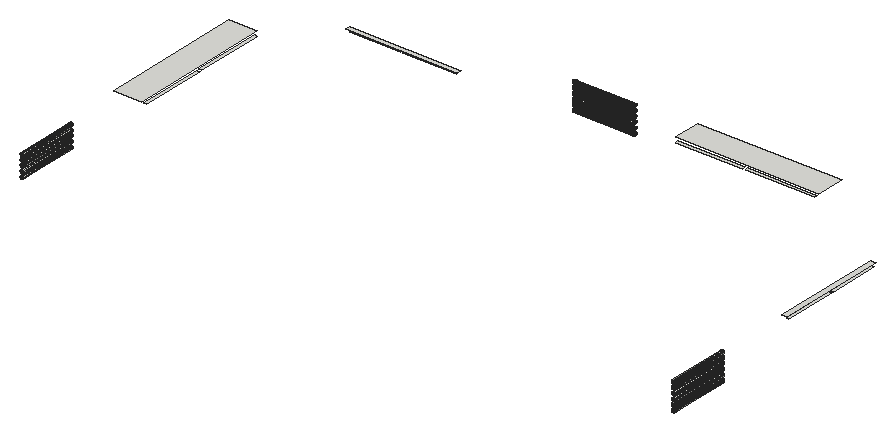
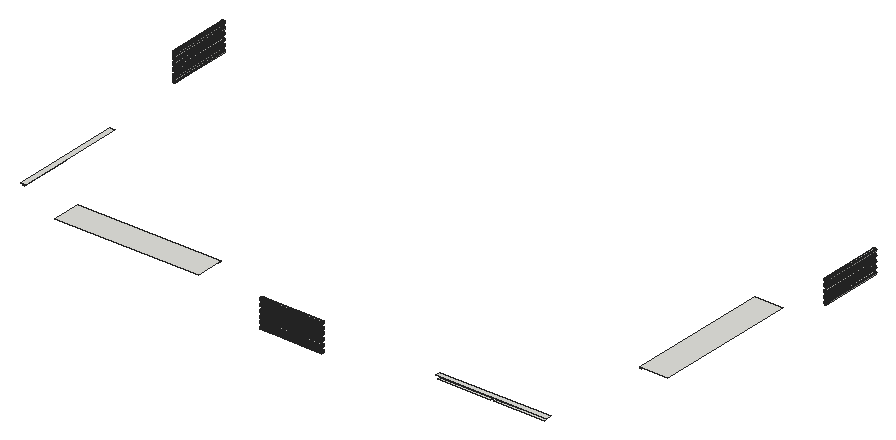
# SketchUp Ruby script. Lengths in inches.
U = 1.inch
M = Sketchup.active_model
def pt(a) = Geom::Point3d.new(a.map { |v| v * U })
def face(e, loops, mat)
  f = e.add_face(loops[0].map { |a| pt(a) })
  loops[1..].each { |l| e.add_face(l.map { |a| pt(a) }).erase! }
  f.material = f.back_material = mat if mat
  f
end
# faces: each face lists its corners as indices into pts; further lists are holes
def faces(e, pts, list, mat = nil) = list.each { |f| face(e, (f[0].is_a?(Array) ? f : [f]).map { |l| l.map { |i| pts[i] } }, mat) }
# xy, xz, yz: faces in a plane at the given z, y or x. An outline is a flat list of corners, or four numbers for a rectangle; further outlines are holes
def ring(l) = l.size == 4 ? [[l[0], l[1]], [l[2], l[1]], [l[2], l[3]], [l[0], l[3]]] : l.each_slice(2).to_a
def flat(e, list, mat, &to3) = list.each { |f| face(e, (f[0].is_a?(Array) ? f : [f]).map { |l| ring(l).map { |u, v| to3.(u, v) } }, mat) }
def xy(e, z, list, mat = nil) = flat(e, list, mat) { |x, y| [x, y, z] }
def xz(e, y, list, mat = nil) = flat(e, list, mat) { |x, z| [x, y, z] }
def yz(e, x, list, mat = nil) = flat(e, list, mat) { |y, z| [x, y, z] }
def lines(e, pts, list) = list.each { |a, b| e.add_line(pt(pts[a]), pt(pts[b])) }
# prism: a flat outline (further loops are holes) pulled along v
def prism(e, loops, v, mat = nil)
  f = face(e, loops, mat); d = Geom::Vector3d.new(v.map { |x| x * U })
  f.pushpull(f.normal.samedirection?(d) ? d.length : -d.length)
end
def box(e, o, s, mat = nil) = prism(e, [[o, [o[0] + s[0], o[1], o[2]], [o[0] + s[0], o[1] + s[1], o[2]], [o[0], o[1] + s[1], o[2]]]], [0, 0, s[2]], mat)
def at(x, y, z, deg = 0) = Geom::Transformation.translation(pt([x, y, z])) * Geom::Transformation.rotation(ORIGIN, Z_AXIS, deg.degrees)
def axes(o, x, y, z) = Geom::Transformation.new([*x, 0, *y, 0, *z, 0, *pt(o).to_a, 1])
def part(name) = M.definitions.add(name)
# library, detail: a bought-in or finely detailed component or shape, given as its bounding box
def library(name, o, s) = part(name).tap { |d| box(d.entities, o, s) }
def detail(e, o, s) = box(e.add_group.entities, o, s)
def put(e, d, t, mat = nil) = e.add_instance(d, t).tap { |i| i.material = mat if mat }
def group(e, t, mat = nil) = e.add_group.tap { |g| g.transformation = t; g.material = mat if mat }.entities
root = M.entities
xy(root,647.61,[[1494,1126.01,1500,1249.86],[1494,1255.86,1500,1373.7],[211.11,1458.8125,328.96,1464.8125],[334.96,1458.8125,458.8,1464.8125]])
xy(root,653.61,[[1488,1120.01,1500,1379.7],[205.11,1452.8125,464.8,1464.8125]])
xy(root,696.625,[[138,949.59,144,1104.875],[138,1110.875,144,1272.16],[984.78,1440.8125,1140.0625,1446.8125],[1146.0625,1440.8125,1307.35,1446.8125]])
xy(root,702.625,[[72,943.59,138,1278.16],[978.78,1446.8125,1313.35,1512.8125]])
p = [[1535.52,886.83,633.14],[1536.47,886.83,633.02],[1536.47,743.45,633.02],[1535.52,743.45,633.14],[1537.43,886.83,633.14],[1537.43,743.45,633.14],
  [697.99,1500.33,633.14],[697.99,1501.28,633.02],[841.36,1501.28,633.02],[841.36,1500.33,633.14],[697.99,1502.24,633.14],[841.36,1502.24,633.14],
  [1534.63,886.83,633.51],[1534.63,743.45,633.51],[1538.32,886.83,633.51],[1538.32,743.45,633.51],[697.99,1499.44,633.51],[841.36,1499.44,633.51],
  [697.99,1503.13,633.51],[841.36,1503.13,633.51],[1533.87,886.83,634.1],[1533.87,743.45,634.1],[1539.08,886.83,634.1],[1539.08,743.45,634.1],
  [697.99,1498.68,634.1],[841.36,1498.68,634.1],[697.99,1503.89,634.1],[841.36,1503.89,634.1],[1533.28,886.83,634.86],[1533.28,743.45,634.86],
  [1539.67,886.83,634.86],[1539.67,743.45,634.86],[697.99,1498.09,634.86],[841.36,1498.09,634.86],[697.99,1504.48,634.86],[841.36,1504.48,634.86],
  [1532.91,886.83,635.75],[1532.91,743.45,635.75],[1540.03,886.83,635.75],[1540.03,743.45,635.75],[697.99,1497.72,635.75],[841.36,1497.72,635.75],
  [697.99,1504.85,635.75],[841.36,1504.85,635.75],[1532.79,886.83,636.7],[1532.79,743.45,636.7],[1540.16,886.83,636.7],[1540.16,743.45,636.7],
  [697.99,1497.6,636.7],[841.36,1497.6,636.7],[697.99,1504.97,636.7],[841.36,1504.97,636.7],[1532.91,886.83,637.66],[1532.91,743.45,637.66],
  [1540.03,886.83,637.66],[1540.03,743.45,637.66],[697.99,1497.72,637.66],[841.36,1497.72,637.66],[697.99,1504.85,637.66],[841.36,1504.85,637.66],
  [1533.28,886.83,638.55],[1533.28,743.45,638.55],[1539.67,886.83,638.55],[1539.67,743.45,638.55],[697.99,1498.09,638.55],[841.36,1498.09,638.55],
  [697.99,1504.48,638.55],[841.36,1504.48,638.55],[1533.87,886.83,639.3125],[1533.87,743.45,639.3125],[1539.08,886.83,639.3125],[1539.08,743.45,639.3125],
  [697.99,1498.68,639.3125],[841.36,1498.68,639.3125],[697.99,1503.89,639.3125],[841.36,1503.89,639.3125],[1534.63,886.83,639.9],[1534.63,743.45,639.9],
  [1538.32,886.83,639.9],[1538.32,743.45,639.9],[697.99,1499.44,639.9],[841.36,1499.44,639.9],[697.99,1503.13,639.9],[841.36,1503.13,639.9],
  [1535.52,886.83,640.27],[1535.52,743.45,640.27],[1537.43,886.83,640.27],[1537.43,743.45,640.27],[697.99,1500.33,640.27],[841.36,1500.33,640.27],
  [697.99,1502.24,640.27],[841.36,1502.24,640.27],[1536.47,886.83,640.39],[1536.47,743.45,640.39],[697.99,1501.28,640.39],[841.36,1501.28,640.39],
  [83.53,662.8,645.02],[82.57,662.8,645.14],[82.57,806.17,645.14],[83.53,806.17,645.02],[84.48,662.8,645.14],[84.48,806.17,645.14],
  [1535.52,886.83,645.14],[1536.47,886.83,645.02],[1536.47,743.45,645.02],[1535.52,743.45,645.14],[1537.43,886.83,645.14],[1537.43,743.45,645.14],
  [697.99,1500.33,645.14],[697.99,1501.28,645.02],[841.36,1501.28,645.02],[841.36,1500.33,645.14],[697.99,1502.24,645.14],[841.36,1502.24,645.14],
  [81.68,662.8,645.51],[81.68,806.17,645.51],[85.37,662.8,645.51],[85.37,806.17,645.51],[1534.63,886.83,645.51],[1534.63,743.45,645.51],
  [1538.32,886.83,645.51],[1538.32,743.45,645.51],[697.99,1499.44,645.51],[841.36,1499.44,645.51],[697.99,1503.13,645.51],[841.36,1503.13,645.51],
  [80.92,662.8,646.1],[80.92,806.17,646.1],[86.13,662.8,646.1],[86.13,806.17,646.1],[1533.87,886.83,646.1],[1533.87,743.45,646.1],
  [1539.08,886.83,646.1],[1539.08,743.45,646.1],[697.99,1498.68,646.1],[841.36,1498.68,646.1],[697.99,1503.89,646.1],[841.36,1503.89,646.1],
  [80.33,662.8,646.86],[80.33,806.17,646.86],[86.72,662.8,646.86],[86.72,806.17,646.86],[1533.28,886.83,646.86],[1533.28,743.45,646.86],
  [1539.67,886.83,646.86],[1539.67,743.45,646.86],[697.99,1498.09,646.86],[841.36,1498.09,646.86],[697.99,1504.48,646.86],[841.36,1504.48,646.86],
  [79.97,662.8,647.75],[79.97,806.17,647.75],[87.09,662.8,647.75],[87.09,806.17,647.75],[1532.91,886.83,647.75],[1532.91,743.45,647.75],
  [1540.03,886.83,647.75],[1540.03,743.45,647.75],[697.99,1497.72,647.75],[841.36,1497.72,647.75],[697.99,1504.85,647.75],[841.36,1504.85,647.75],
  [79.84,662.8,648.7],[79.84,806.17,648.7],[87.21,662.8,648.7],[87.21,806.17,648.7],[1532.79,886.83,648.7],[1532.79,743.45,648.7],
  [1540.16,886.83,648.7],[1540.16,743.45,648.7],[697.99,1497.6,648.7],[841.36,1497.6,648.7],[697.99,1504.97,648.7],[841.36,1504.97,648.7],
  [79.97,662.8,649.66],[79.97,806.17,649.66],[87.09,662.8,649.66],[87.09,806.17,649.66],[1532.91,886.83,649.66],[1532.91,743.45,649.66],
  [1540.03,886.83,649.66],[1540.03,743.45,649.66],[697.99,1497.72,649.66],[841.36,1497.72,649.66],[697.99,1504.85,649.66],[841.36,1504.85,649.66],
  [80.33,662.8,650.55],[80.33,806.17,650.55],[86.72,662.8,650.55],[86.72,806.17,650.55],[1533.28,886.83,650.55],[1533.28,743.45,650.55],
  [1539.67,886.83,650.55],[1539.67,743.45,650.55],[697.99,1498.09,650.55],[841.36,1498.09,650.55],[697.99,1504.48,650.55],[841.36,1504.48,650.55],
  [80.92,662.8,651.3125],[80.92,806.17,651.3125],[86.13,662.8,651.3125],[86.13,806.17,651.3125],[1533.87,886.83,651.3125],[1533.87,743.45,651.3125],
  [1539.08,886.83,651.3125],[1539.08,743.45,651.3125],[697.99,1498.68,651.3125],[841.36,1498.68,651.3125],[697.99,1503.89,651.3125],[841.36,1503.89,651.3125],
  [81.68,662.8,651.9],[81.68,806.17,651.9],[85.37,662.8,651.9],[85.37,806.17,651.9],[1534.63,886.83,651.9],[1534.63,743.45,651.9],
  [1538.32,886.83,651.9],[1538.32,743.45,651.9],[697.99,1499.44,651.9],[841.36,1499.44,651.9],[697.99,1503.13,651.9],[841.36,1503.13,651.9],
  [82.57,662.8,652.27],[82.57,806.17,652.27],[84.48,662.8,652.27],[84.48,806.17,652.27],[1535.52,886.83,652.27],[1535.52,743.45,652.27],
  [1537.43,886.83,652.27],[1537.43,743.45,652.27],[697.99,1500.33,652.27],[841.36,1500.33,652.27],[697.99,1502.24,652.27],[841.36,1502.24,652.27],
  [83.53,662.8,652.39],[83.53,806.17,652.39],[1536.47,886.83,652.39],[1536.47,743.45,652.39],[697.99,1501.28,652.39],[841.36,1501.28,652.39],
  [83.53,662.8,657.02],[82.57,662.8,657.14],[82.57,806.17,657.14],[83.53,806.17,657.02],[84.48,662.8,657.14],[84.48,806.17,657.14],
  [1535.52,886.83,657.14],[1536.47,886.83,657.02],[1536.47,743.45,657.02],[1535.52,743.45,657.14],[1537.43,886.83,657.14],[1537.43,743.45,657.14],
  [697.99,1500.33,657.14],[697.99,1501.28,657.02],[841.36,1501.28,657.02],[841.36,1500.33,657.14],[697.99,1502.24,657.14],[841.36,1502.24,657.14],
  [81.68,662.8,657.51],[81.68,806.17,657.51],[85.37,662.8,657.51],[85.37,806.17,657.51],[1534.63,886.83,657.51],[1534.63,743.45,657.51],
  [1538.32,886.83,657.51],[1538.32,743.45,657.51],[697.99,1499.44,657.51],[841.36,1499.44,657.51],[697.99,1503.13,657.51],[841.36,1503.13,657.51],
  [80.92,662.8,658.1],[80.92,806.17,658.1],[86.13,662.8,658.1],[86.13,806.17,658.1],[1533.87,886.83,658.1],[1533.87,743.45,658.1],
  [1539.08,886.83,658.1],[1539.08,743.45,658.1],[697.99,1498.68,658.1],[841.36,1498.68,658.1],[697.99,1503.89,658.1],[841.36,1503.89,658.1],
  [80.33,662.8,658.86],[80.33,806.17,658.86],[86.72,662.8,658.86],[86.72,806.17,658.86],[1533.28,886.83,658.86],[1533.28,743.45,658.86],
  [1539.67,886.83,658.86],[1539.67,743.45,658.86],[697.99,1498.09,658.86],[841.36,1498.09,658.86],[697.99,1504.48,658.86],[841.36,1504.48,658.86],
  [79.97,662.8,659.75],[79.97,806.17,659.75],[87.09,662.8,659.75],[87.09,806.17,659.75],[1532.91,886.83,659.75],[1532.91,743.45,659.75],
  [1540.03,886.83,659.75],[1540.03,743.45,659.75],[697.99,1497.72,659.75],[841.36,1497.72,659.75],[697.99,1504.85,659.75],[841.36,1504.85,659.75],
  [79.84,662.8,660.7],[79.84,806.17,660.7],[87.21,662.8,660.7],[87.21,806.17,660.7],[1532.79,886.83,660.7],[1532.79,743.45,660.7],
  [1540.16,886.83,660.7],[1540.16,743.45,660.7],[697.99,1497.6,660.7],[841.36,1497.6,660.7],[697.99,1504.97,660.7],[841.36,1504.97,660.7],
  [79.97,662.8,661.66],[79.97,806.17,661.66],[87.09,662.8,661.66],[87.09,806.17,661.66],[1532.91,886.83,661.66],[1532.91,743.45,661.66],
  [1540.03,886.83,661.66],[1540.03,743.45,661.66],[697.99,1497.72,661.66],[841.36,1497.72,661.66],[697.99,1504.85,661.66],[841.36,1504.85,661.66],
  [80.33,662.8,662.55],[80.33,806.17,662.55],[86.72,662.8,662.55],[86.72,806.17,662.55],[1533.28,886.83,662.55],[1533.28,743.45,662.55],
  [1539.67,886.83,662.55],[1539.67,743.45,662.55],[697.99,1498.09,662.55],[841.36,1498.09,662.55],[697.99,1504.48,662.55],[841.36,1504.48,662.55],
  [80.92,662.8,663.3125],[80.92,806.17,663.3125],[86.13,662.8,663.3125],[86.13,806.17,663.3125],[1533.87,886.83,663.3125],[1533.87,743.45,663.3125],
  [1539.08,886.83,663.3125],[1539.08,743.45,663.3125],[697.99,1498.68,663.3125],[841.36,1498.68,663.3125],[697.99,1503.89,663.3125],[841.36,1503.89,663.3125],
  [81.68,662.8,663.9],[81.68,806.17,663.9],[85.37,662.8,663.9],[85.37,806.17,663.9],[1534.63,886.83,663.9],[1534.63,743.45,663.9],
  [1538.32,886.83,663.9],[1538.32,743.45,663.9],[697.99,1499.44,663.9],[841.36,1499.44,663.9],[697.99,1503.13,663.9],[841.36,1503.13,663.9],
  [82.57,662.8,664.27],[82.57,806.17,664.27],[84.48,662.8,664.27],[84.48,806.17,664.27],[1535.52,886.83,664.27],[1535.52,743.45,664.27],
  [1537.43,886.83,664.27],[1537.43,743.45,664.27],[697.99,1500.33,664.27],[841.36,1500.33,664.27],[697.99,1502.24,664.27],[841.36,1502.24,664.27],
  [83.53,662.8,664.39],[83.53,806.17,664.39],[1536.47,886.83,664.39],[1536.47,743.45,664.39],[697.99,1501.28,664.39],[841.36,1501.28,664.39],
  [83.53,662.8,669.02],[82.57,662.8,669.14],[82.57,806.17,669.14],[83.53,806.17,669.02],[84.48,662.8,669.14],[84.48,806.17,669.14],
  [1535.52,886.83,669.14],[1536.47,886.83,669.02],[1536.47,743.45,669.02],[1535.52,743.45,669.14],[1537.43,886.83,669.14],[1537.43,743.45,669.14],
  [697.99,1500.33,669.14],[697.99,1501.28,669.02],[841.36,1501.28,669.02],[841.36,1500.33,669.14],[697.99,1502.24,669.14],[841.36,1502.24,669.14],
  [81.68,662.8,669.51],[81.68,806.17,669.51],[85.37,662.8,669.51],[85.37,806.17,669.51],[1534.63,886.83,669.51],[1534.63,743.45,669.51],
  [1538.32,886.83,669.51],[1538.32,743.45,669.51],[697.99,1499.44,669.51],[841.36,1499.44,669.51],[697.99,1503.13,669.51],[841.36,1503.13,669.51],
  [80.92,662.8,670.1],[80.92,806.17,670.1],[86.13,662.8,670.1],[86.13,806.17,670.1],[1533.87,886.83,670.1],[1533.87,743.45,670.1],
  [1539.08,886.83,670.1],[1539.08,743.45,670.1],[697.99,1498.68,670.1],[841.36,1498.68,670.1],[697.99,1503.89,670.1],[841.36,1503.89,670.1],
  [80.33,662.8,670.86],[80.33,806.17,670.86],[86.72,662.8,670.86],[86.72,806.17,670.86],[1533.28,886.83,670.86],[1533.28,743.45,670.86],
  [1539.67,886.83,670.86],[1539.67,743.45,670.86],[697.99,1498.09,670.86],[841.36,1498.09,670.86],[697.99,1504.48,670.86],[841.36,1504.48,670.86],
  [79.97,662.8,671.75],[79.97,806.17,671.75],[87.09,662.8,671.75],[87.09,806.17,671.75],[1532.91,886.83,671.75],[1532.91,743.45,671.75],
  [1540.03,886.83,671.75],[1540.03,743.45,671.75],[697.99,1497.72,671.75],[841.36,1497.72,671.75],[697.99,1504.85,671.75],[841.36,1504.85,671.75],
  [79.84,662.8,672.7],[79.84,806.17,672.7],[87.21,662.8,672.7],[87.21,806.17,672.7],[1532.79,886.83,672.7],[1532.79,743.45,672.7],
  [1540.16,886.83,672.7],[1540.16,743.45,672.7],[697.99,1497.6,672.7],[841.36,1497.6,672.7],[697.99,1504.97,672.7],[841.36,1504.97,672.7],
  [79.97,662.8,673.66],[79.97,806.17,673.66],[87.09,662.8,673.66],[87.09,806.17,673.66],[1532.91,886.83,673.66],[1532.91,743.45,673.66],
  [1540.03,886.83,673.66],[1540.03,743.45,673.66],[697.99,1497.72,673.66],[841.36,1497.72,673.66],[697.99,1504.85,673.66],[841.36,1504.85,673.66],
  [80.33,662.8,674.55],[80.33,806.17,674.55],[86.72,662.8,674.55],[86.72,806.17,674.55],[1533.28,886.83,674.55],[1533.28,743.45,674.55],
  [1539.67,886.83,674.55],[1539.67,743.45,674.55],[697.99,1498.09,674.55],[841.36,1498.09,674.55],[697.99,1504.48,674.55],[841.36,1504.48,674.55],
  [80.92,662.8,675.3125],[80.92,806.17,675.3125],[86.13,662.8,675.3125],[86.13,806.17,675.3125],[1533.87,886.83,675.3125],[1533.87,743.45,675.3125],
  [1539.08,886.83,675.3125],[1539.08,743.45,675.3125],[697.99,1498.68,675.3125],[841.36,1498.68,675.3125],[697.99,1503.89,675.3125],[841.36,1503.89,675.3125],
  [81.68,662.8,675.9],[81.68,806.17,675.9],[85.37,662.8,675.9],[85.37,806.17,675.9],[1534.63,886.83,675.9],[1534.63,743.45,675.9],
  [1538.32,886.83,675.9],[1538.32,743.45,675.9],[697.99,1499.44,675.9],[841.36,1499.44,675.9],[697.99,1503.13,675.9],[841.36,1503.13,675.9],
  [82.57,662.8,676.27],[82.57,806.17,676.27],[84.48,662.8,676.27],[84.48,806.17,676.27],[1535.52,886.83,676.27],[1535.52,743.45,676.27],
  [1537.43,886.83,676.27],[1537.43,743.45,676.27],[697.99,1500.33,676.27],[841.36,1500.33,676.27],[697.99,1502.24,676.27],[841.36,1502.24,676.27],
  [83.53,662.8,676.39],[83.53,806.17,676.39],[1536.47,886.83,676.39],[1536.47,743.45,676.39],[697.99,1501.28,676.39],[841.36,1501.28,676.39],
  [83.53,662.8,681.02],[82.57,662.8,681.14],[82.57,806.17,681.14],[83.53,806.17,681.02],[84.48,662.8,681.14],[84.48,806.17,681.14],
  [1535.52,886.83,681.14],[1536.47,886.83,681.02],[1536.47,743.45,681.02],[1535.52,743.45,681.14],[1537.43,886.83,681.14],[1537.43,743.45,681.14],
  [697.99,1500.33,681.14],[697.99,1501.28,681.02],[841.36,1501.28,681.02],[841.36,1500.33,681.14],[697.99,1502.24,681.14],[841.36,1502.24,681.14],
  [81.68,662.8,681.51],[81.68,806.17,681.51],[85.37,662.8,681.51],[85.37,806.17,681.51],[1534.63,886.83,681.51],[1534.63,743.45,681.51],
  [1538.32,886.83,681.51],[1538.32,743.45,681.51],[697.99,1499.44,681.51],[841.36,1499.44,681.51],[697.99,1503.13,681.51],[841.36,1503.13,681.51],
  [80.92,662.8,682.1],[80.92,806.17,682.1],[86.13,662.8,682.1],[86.13,806.17,682.1],[1533.87,886.83,682.1],[1533.87,743.45,682.1],
  [1539.08,886.83,682.1],[1539.08,743.45,682.1],[697.99,1498.68,682.1],[841.36,1498.68,682.1],[697.99,1503.89,682.1],[841.36,1503.89,682.1],
  [80.33,662.8,682.86],[80.33,806.17,682.86],[86.72,662.8,682.86],[86.72,806.17,682.86],[1533.28,886.83,682.86],[1533.28,743.45,682.86],
  [1539.67,886.83,682.86],[1539.67,743.45,682.86],[697.99,1498.09,682.86],[841.36,1498.09,682.86],[697.99,1504.48,682.86],[841.36,1504.48,682.86],
  [79.97,662.8,683.75],[79.97,806.17,683.75],[87.09,662.8,683.75],[87.09,806.17,683.75],[1532.91,886.83,683.75],[1532.91,743.45,683.75],
  [1540.03,886.83,683.75],[1540.03,743.45,683.75],[697.99,1497.72,683.75],[841.36,1497.72,683.75],[697.99,1504.85,683.75],[841.36,1504.85,683.75],
  [79.84,662.8,684.7],[79.84,806.17,684.7],[87.21,662.8,684.7],[87.21,806.17,684.7],[1532.79,886.83,684.7],[1532.79,743.45,684.7],
  [1540.16,886.83,684.7],[1540.16,743.45,684.7],[697.99,1497.6,684.7],[841.36,1497.6,684.7],[697.99,1504.97,684.7],[841.36,1504.97,684.7],
  [79.97,662.8,685.66],[79.97,806.17,685.66],[87.09,662.8,685.66],[87.09,806.17,685.66],[1532.91,886.83,685.66],[1532.91,743.45,685.66],
  [1540.03,886.83,685.66],[1540.03,743.45,685.66],[697.99,1497.72,685.66],[841.36,1497.72,685.66],[697.99,1504.85,685.66],[841.36,1504.85,685.66],
  [80.33,662.8,686.55],[80.33,806.17,686.55],[86.72,662.8,686.55],[86.72,806.17,686.55],[1533.28,886.83,686.55],[1533.28,743.45,686.55],
  [1539.67,886.83,686.55],[1539.67,743.45,686.55],[697.99,1498.09,686.55],[841.36,1498.09,686.55],[697.99,1504.48,686.55],[841.36,1504.48,686.55],
  [80.92,662.8,687.3125],[80.92,806.17,687.3125],[86.13,662.8,687.3125],[86.13,806.17,687.3125],[1533.87,886.83,687.3125],[1533.87,743.45,687.3125],
  [1539.08,886.83,687.3125],[1539.08,743.45,687.3125],[697.99,1498.68,687.3125],[841.36,1498.68,687.3125],[697.99,1503.89,687.3125],[841.36,1503.89,687.3125],
  [81.68,662.8,687.9],[81.68,806.17,687.9],[85.37,662.8,687.9],[85.37,806.17,687.9],[1534.63,886.83,687.9],[1534.63,743.45,687.9],
  [1538.32,886.83,687.9],[1538.32,743.45,687.9],[697.99,1499.44,687.9],[841.36,1499.44,687.9],[697.99,1503.13,687.9],[841.36,1503.13,687.9],
  [82.57,662.8,688.27],[82.57,806.17,688.27],[84.48,662.8,688.27],[84.48,806.17,688.27],[1535.52,886.83,688.27],[1535.52,743.45,688.27],
  [1537.43,886.83,688.27],[1537.43,743.45,688.27],[697.99,1500.33,688.27],[841.36,1500.33,688.27],[697.99,1502.24,688.27],[841.36,1502.24,688.27],
  [83.53,662.8,688.39],[83.53,806.17,688.39],[1536.47,886.83,688.39],[1536.47,743.45,688.39],[697.99,1501.28,688.39],[841.36,1501.28,688.39],
  [83.53,662.8,693.02],[82.57,662.8,693.14],[82.57,806.17,693.14],[83.53,806.17,693.02],[84.48,662.8,693.14],[84.48,806.17,693.14],
  [1535.52,886.83,693.14],[1536.47,886.83,693.02],[1536.47,743.45,693.02],[1535.52,743.45,693.14],[1537.43,886.83,693.14],[1537.43,743.45,693.14],
  [697.99,1500.33,693.14],[697.99,1501.28,693.02],[841.36,1501.28,693.02],[841.36,1500.33,693.14],[697.99,1502.24,693.14],[841.36,1502.24,693.14],
  [81.68,662.8,693.51],[81.68,806.17,693.51],[85.37,662.8,693.51],[85.37,806.17,693.51],[1534.63,886.83,693.51],[1534.63,743.45,693.51],
  [1538.32,886.83,693.51],[1538.32,743.45,693.51],[697.99,1499.44,693.51],[841.36,1499.44,693.51],[697.99,1503.13,693.51],[841.36,1503.13,693.51],
  [80.92,662.8,694.1],[80.92,806.17,694.1],[86.13,662.8,694.1],[86.13,806.17,694.1],[1533.87,886.83,694.1],[1533.87,743.45,694.1],
  [1539.08,886.83,694.1],[1539.08,743.45,694.1],[697.99,1498.68,694.1],[841.36,1498.68,694.1],[697.99,1503.89,694.1],[841.36,1503.89,694.1],
  [80.33,662.8,694.86],[80.33,806.17,694.86],[86.72,662.8,694.86],[86.72,806.17,694.86],[1533.28,886.83,694.86],[1533.28,743.45,694.86],
  [1539.67,886.83,694.86],[1539.67,743.45,694.86],[697.99,1498.09,694.86],[841.36,1498.09,694.86],[697.99,1504.48,694.86],[841.36,1504.48,694.86],
  [79.97,662.8,695.75],[79.97,806.17,695.75],[87.09,662.8,695.75],[87.09,806.17,695.75],[1532.91,886.83,695.75],[1532.91,743.45,695.75],
  [1540.03,886.83,695.75],[1540.03,743.45,695.75],[697.99,1497.72,695.75],[841.36,1497.72,695.75],[697.99,1504.85,695.75],[841.36,1504.85,695.75],
  [79.84,662.8,696.7],[79.84,806.17,696.7],[87.21,662.8,696.7],[87.21,806.17,696.7],[1532.79,886.83,696.7],[1532.79,743.45,696.7],
  [1540.16,886.83,696.7],[1540.16,743.45,696.7],[697.99,1497.6,696.7],[841.36,1497.6,696.7],[697.99,1504.97,696.7],[841.36,1504.97,696.7],
  [79.97,662.8,697.66],[79.97,806.17,697.66],[87.09,662.8,697.66],[87.09,806.17,697.66],[1532.91,886.83,697.66],[1532.91,743.45,697.66],
  [1540.03,886.83,697.66],[1540.03,743.45,697.66],[697.99,1497.72,697.66],[841.36,1497.72,697.66],[697.99,1504.85,697.66],[841.36,1504.85,697.66],
  [80.33,662.8,698.55],[80.33,806.17,698.55],[86.72,662.8,698.55],[86.72,806.17,698.55],[1533.28,886.83,698.55],[1533.28,743.45,698.55],
  [1539.67,886.83,698.55],[1539.67,743.45,698.55],[697.99,1498.09,698.55],[841.36,1498.09,698.55],[697.99,1504.48,698.55],[841.36,1504.48,698.55],
  [80.92,662.8,699.3125],[80.92,806.17,699.3125],[86.13,662.8,699.3125],[86.13,806.17,699.3125],[1533.87,886.83,699.3125],[1533.87,743.45,699.3125],
  [1539.08,886.83,699.3125],[1539.08,743.45,699.3125],[697.99,1498.68,699.3125],[841.36,1498.68,699.3125],[697.99,1503.89,699.3125],[841.36,1503.89,699.3125],
  [81.68,662.8,699.9],[81.68,806.17,699.9],[85.37,662.8,699.9],[85.37,806.17,699.9],[1534.63,886.83,699.9],[1534.63,743.45,699.9],
  [1538.32,886.83,699.9],[1538.32,743.45,699.9],[697.99,1499.44,699.9],[841.36,1499.44,699.9],[697.99,1503.13,699.9],[841.36,1503.13,699.9],
  [82.57,662.8,700.27],[82.57,806.17,700.27],[84.48,662.8,700.27],[84.48,806.17,700.27],[1535.52,886.83,700.27],[1535.52,743.45,700.27],
  [1537.43,886.83,700.27],[1537.43,743.45,700.27],[697.99,1500.33,700.27],[841.36,1500.33,700.27],[697.99,1502.24,700.27],[841.36,1502.24,700.27],
  [83.53,662.8,700.39],[83.53,806.17,700.39],[1536.47,886.83,700.39],[1536.47,743.45,700.39],[697.99,1501.28,700.39],[841.36,1501.28,700.39]]
faces(root,p,[[0,1,2,3],[1,4,5,2],[6,7,8,9],[7,10,11,8],[12,0,3,13],[4,14,15,5],[16,6,9,17],[10,18,19,11],
  [20,12,13,21],[14,22,23,15],[24,16,17,25],[18,26,27,19],[28,20,21,29],[22,30,31,23],[32,24,25,33],[26,34,35,27],
  [36,28,29,37],[30,38,39,31],[40,32,33,41],[34,42,43,35],[44,36,37,45],[38,46,47,39],[48,40,41,49],[42,50,51,43],
  [52,44,45,53],[46,54,55,47],[56,48,49,57],[50,58,59,51],[60,52,53,61],[54,62,63,55],[64,56,57,65],[58,66,67,59],
  [68,60,61,69],[62,70,71,63],[72,64,65,73],[66,74,75,67],[76,68,69,77],[70,78,79,71],[80,72,73,81],[74,82,83,75],
  [84,76,77,85],[78,86,87,79],[88,80,81,89],[82,90,91,83],[92,84,85,93],[86,92,93,87],[94,88,89,95],[90,94,95,91],
  [96,97,98,99],[100,96,99,101],[102,103,104,105],[103,106,107,104],[108,109,110,111],[109,112,113,110],[97,114,115,98],[116,100,101,117],
  [118,102,105,119],[106,120,121,107],[122,108,111,123],[112,124,125,113],[114,126,127,115],[128,116,117,129],[130,118,119,131],[120,132,133,121],
  [134,122,123,135],[124,136,137,125],[126,138,139,127],[140,128,129,141],[142,130,131,143],[132,144,145,133],[146,134,135,147],[136,148,149,137],
  [138,150,151,139],[152,140,141,153],[154,142,143,155],[144,156,157,145],[158,146,147,159],[148,160,161,149],[150,162,163,151],[164,152,153,165],
  [166,154,155,167],[156,168,169,157],[170,158,159,171],[160,172,173,161],[162,174,175,163],[176,164,165,177],[178,166,167,179],[168,180,181,169],
  [182,170,171,183],[172,184,185,173],[174,186,187,175],[188,176,177,189],[190,178,179,191],[180,192,193,181],[194,182,183,195],[184,196,197,185],
  [186,198,199,187],[200,188,189,201],[202,190,191,203],[192,204,205,193],[206,194,195,207],[196,208,209,197],[198,210,211,199],[212,200,201,213],
  [214,202,203,215],[204,216,217,205],[218,206,207,219],[208,220,221,209],[210,222,223,211],[224,212,213,225],[226,214,215,227],[216,228,229,217],
  [230,218,219,231],[220,232,233,221],[222,234,235,223],[234,224,225,235],[236,226,227,237],[228,236,237,229],[238,230,231,239],[232,238,239,233],
  [240,241,242,243],[244,240,243,245],[246,247,248,249],[247,250,251,248],[252,253,254,255],[253,256,257,254],[241,258,259,242],[260,244,245,261],
  [262,246,249,263],[250,264,265,251],[266,252,255,267],[256,268,269,257],[258,270,271,259],[272,260,261,273],[274,262,263,275],[264,276,277,265],
  [278,266,267,279],[268,280,281,269],[270,282,283,271],[284,272,273,285],[286,274,275,287],[276,288,289,277],[290,278,279,291],[280,292,293,281],
  [282,294,295,283],[296,284,285,297],[298,286,287,299],[288,300,301,289],[302,290,291,303],[292,304,305,293],[294,306,307,295],[308,296,297,309],
  [310,298,299,311],[300,312,313,301],[314,302,303,315],[304,316,317,305],[306,318,319,307],[320,308,309,321],[322,310,311,323],[312,324,325,313],
  [326,314,315,327],[316,328,329,317],[318,330,331,319],[332,320,321,333],[334,322,323,335],[324,336,337,325],[338,326,327,339],[328,340,341,329],
  [330,342,343,331],[344,332,333,345],[346,334,335,347],[336,348,349,337],[350,338,339,351],[340,352,353,341],[342,354,355,343],[356,344,345,357],
  [358,346,347,359],[348,360,361,349],[362,350,351,363],[352,364,365,353],[354,366,367,355],[368,356,357,369],[370,358,359,371],[360,372,373,361],
  [374,362,363,375],[364,376,377,365],[366,378,379,367],[378,368,369,379],[380,370,371,381],[372,380,381,373],[382,374,375,383],[376,382,383,377],
  [384,385,386,387],[388,384,387,389],[390,391,392,393],[391,394,395,392],[396,397,398,399],[397,400,401,398],[385,402,403,386],[404,388,389,405],
  [406,390,393,407],[394,408,409,395],[410,396,399,411],[400,412,413,401],[402,414,415,403],[416,404,405,417],[418,406,407,419],[408,420,421,409],
  [422,410,411,423],[412,424,425,413],[414,426,427,415],[428,416,417,429],[430,418,419,431],[420,432,433,421],[434,422,423,435],[424,436,437,425],
  [426,438,439,427],[440,428,429,441],[442,430,431,443],[432,444,445,433],[446,434,435,447],[436,448,449,437],[438,450,451,439],[452,440,441,453],
  [454,442,443,455],[444,456,457,445],[458,446,447,459],[448,460,461,449],[450,462,463,451],[464,452,453,465],[466,454,455,467],[456,468,469,457],
  [470,458,459,471],[460,472,473,461],[462,474,475,463],[476,464,465,477],[478,466,467,479],[468,480,481,469],[482,470,471,483],[472,484,485,473],
  [474,486,487,475],[488,476,477,489],[490,478,479,491],[480,492,493,481],[494,482,483,495],[484,496,497,485],[486,498,499,487],[500,488,489,501],
  [502,490,491,503],[492,504,505,493],[506,494,495,507],[496,508,509,497],[498,510,511,499],[512,500,501,513],[514,502,503,515],[504,516,517,505],
  [518,506,507,519],[508,520,521,509],[510,522,523,511],[522,512,513,523],[524,514,515,525],[516,524,525,517],[526,518,519,527],[520,526,527,521],
  [528,529,530,531],[532,528,531,533],[534,535,536,537],[535,538,539,536],[540,541,542,543],[541,544,545,542],[529,546,547,530],[548,532,533,549],
  [550,534,537,551],[538,552,553,539],[554,540,543,555],[544,556,557,545],[546,558,559,547],[560,548,549,561],[562,550,551,563],[552,564,565,553],
  [566,554,555,567],[556,568,569,557],[558,570,571,559],[572,560,561,573],[574,562,563,575],[564,576,577,565],[578,566,567,579],[568,580,581,569],
  [570,582,583,571],[584,572,573,585],[586,574,575,587],[576,588,589,577],[590,578,579,591],[580,592,593,581],[582,594,595,583],[596,584,585,597],
  [598,586,587,599],[588,600,601,589],[602,590,591,603],[592,604,605,593],[594,606,607,595],[608,596,597,609],[610,598,599,611],[600,612,613,601],
  [614,602,603,615],[604,616,617,605],[606,618,619,607],[620,608,609,621],[622,610,611,623],[612,624,625,613],[626,614,615,627],[616,628,629,617],
  [618,630,631,619],[632,620,621,633],[634,622,623,635],[624,636,637,625],[638,626,627,639],[628,640,641,629],[630,642,643,631],[644,632,633,645],
  [646,634,635,647],[636,648,649,637],[650,638,639,651],[640,652,653,641],[642,654,655,643],[656,644,645,657],[658,646,647,659],[648,660,661,649],
  [662,650,651,663],[652,664,665,653],[654,666,667,655],[666,656,657,667],[668,658,659,669],[660,668,669,661],[670,662,663,671],[664,670,671,665],
  [672,673,674,675],[676,672,675,677],[678,679,680,681],[679,682,683,680],[684,685,686,687],[685,688,689,686],[673,690,691,674],[692,676,677,693],
  [694,678,681,695],[682,696,697,683],[698,684,687,699],[688,700,701,689],[690,702,703,691],[704,692,693,705],[706,694,695,707],[696,708,709,697],
  [710,698,699,711],[700,712,713,701],[702,714,715,703],[716,704,705,717],[718,706,707,719],[708,720,721,709],[722,710,711,723],[712,724,725,713],
  [714,726,727,715],[728,716,717,729],[730,718,719,731],[720,732,733,721],[734,722,723,735],[724,736,737,725],[726,738,739,727],[740,728,729,741],
  [742,730,731,743],[732,744,745,733],[746,734,735,747],[736,748,749,737],[738,750,751,739],[752,740,741,753],[754,742,743,755],[744,756,757,745],
  [758,746,747,759],[748,760,761,749],[750,762,763,751],[764,752,753,765],[766,754,755,767],[756,768,769,757],[770,758,759,771],[760,772,773,761],
  [762,774,775,763],[776,764,765,777],[778,766,767,779],[768,780,781,769],[782,770,771,783],[772,784,785,773],[774,786,787,775],[788,776,777,789],
  [790,778,779,791],[780,792,793,781],[794,782,783,795],[784,796,797,785],[786,798,799,787],[800,788,789,801],[802,790,791,803],[792,804,805,793],
  [806,794,795,807],[796,808,809,797],[798,810,811,799],[810,800,801,811],[812,802,803,813],[804,812,813,805],[814,806,807,815],[808,814,815,809]])
